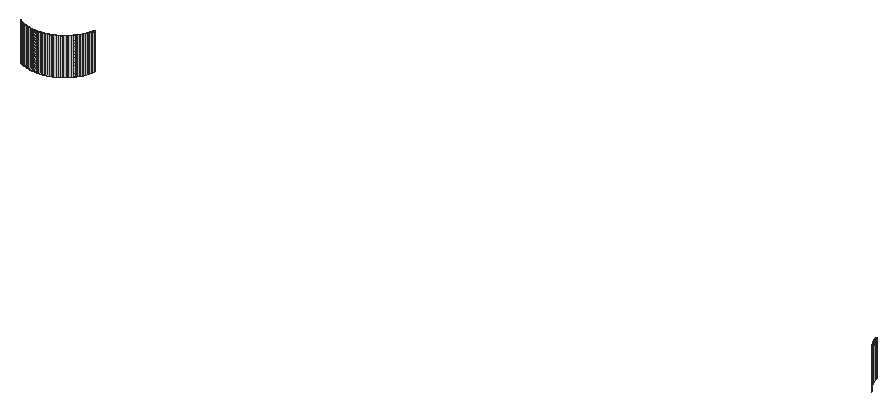
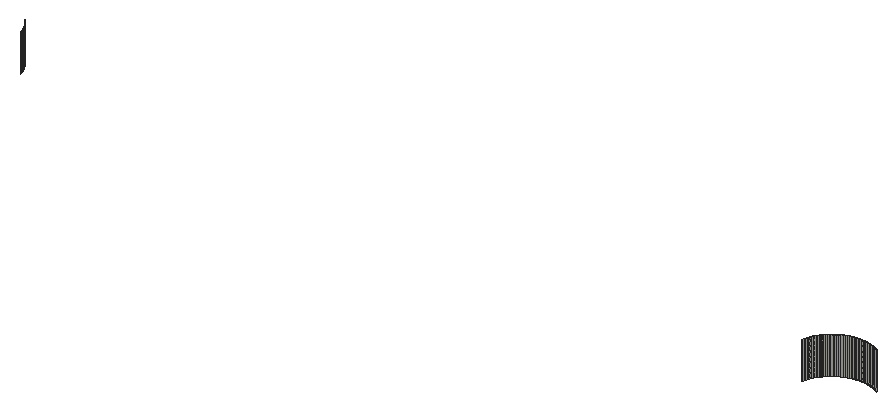
# SketchUp Ruby script. Lengths in inches.
U = 1.inch
M = Sketchup.active_model
def pt(a) = Geom::Point3d.new(a.map { |v| v * U })
def face(e, loops, mat)
  f = e.add_face(loops[0].map { |a| pt(a) })
  loops[1..].each { |l| e.add_face(l.map { |a| pt(a) }).erase! }
  f.material = f.back_material = mat if mat
  f
end
# faces: each face lists its corners as indices into pts; further lists are holes
def faces(e, pts, list, mat = nil) = list.each { |f| face(e, (f[0].is_a?(Array) ? f : [f]).map { |l| l.map { |i| pts[i] } }, mat) }
# xy, xz, yz: faces in a plane at the given z, y or x. An outline is a flat list of corners, or four numbers for a rectangle; further outlines are holes
def ring(l) = l.size == 4 ? [[l[0], l[1]], [l[2], l[1]], [l[2], l[3]], [l[0], l[3]]] : l.each_slice(2).to_a
def flat(e, list, mat, &to3) = list.each { |f| face(e, (f[0].is_a?(Array) ? f : [f]).map { |l| ring(l).map { |u, v| to3.(u, v) } }, mat) }
def xy(e, z, list, mat = nil) = flat(e, list, mat) { |x, y| [x, y, z] }
def xz(e, y, list, mat = nil) = flat(e, list, mat) { |x, z| [x, y, z] }
def yz(e, x, list, mat = nil) = flat(e, list, mat) { |y, z| [x, y, z] }
def lines(e, pts, list) = list.each { |a, b| e.add_line(pt(pts[a]), pt(pts[b])) }
# prism: a flat outline (further loops are holes) pulled along v
def prism(e, loops, v, mat = nil)
  f = face(e, loops, mat); d = Geom::Vector3d.new(v.map { |x| x * U })
  f.pushpull(f.normal.samedirection?(d) ? d.length : -d.length)
end
def box(e, o, s, mat = nil) = prism(e, [[o, [o[0] + s[0], o[1], o[2]], [o[0] + s[0], o[1] + s[1], o[2]], [o[0], o[1] + s[1], o[2]]]], [0, 0, s[2]], mat)
def at(x, y, z, deg = 0) = Geom::Transformation.translation(pt([x, y, z])) * Geom::Transformation.rotation(ORIGIN, Z_AXIS, deg.degrees)
def axes(o, x, y, z) = Geom::Transformation.new([*x, 0, *y, 0, *z, 0, *pt(o).to_a, 1])
def part(name) = M.definitions.add(name)
# library, detail: a bought-in or finely detailed component or shape, given as its bounding box
def library(name, o, s) = part(name).tap { |d| box(d.entities, o, s) }
def detail(e, o, s) = box(e.add_group.entities, o, s)
def put(e, d, t, mat = nil) = e.add_instance(d, t).tap { |i| i.material = mat if mat }
def group(e, t, mat = nil) = e.add_group.tap { |g| g.transformation = t; g.material = mat if mat }.entities
root = M.entities
xz(root,249,[[182.84,348,182.92,351],[182.92,348,183,351],[183,348,183.08,351],[183.08,348,183.16,351]])
p = [[182.53,249.04,348],[182.45,249.05,348],[182.45,249.05,351],[182.53,249.04,351],[182.61,249.03,348],[182.61,249.03,351],
  [182.6875,249.02,348],[182.6875,249.02,351],[182.76,249.01,348],[182.76,249.01,351],[182.84,249,348],[182.84,249,351],
  [183.24,249.01,348],[183.16,249,348],[183.16,249,351],[183.24,249.01,351],[183.3125,249.02,348],[183.3125,249.02,351],
  [183.39,249.03,348],[183.39,249.03,351],[183.47,249.04,348],[183.47,249.04,351],[183.55,249.05,348],[183.55,249.05,351],
  [182.07,249.15,348],[182,249.17,348],[182,249.17,351],[182.07,249.15,351],[182.15,249.125,348],[182.15,249.125,351],
  [182.22,249.1,348],[182.22,249.1,351],[182.3,249.08,348],[182.3,249.08,351],[182.375,249.07,348],[182.375,249.07,351],
  [183.625,249.07,348],[183.625,249.07,351],[183.7,249.08,348],[183.7,249.08,351],[183.78,249.1,348],[183.78,249.1,351],
  [183.85,249.125,348],[183.85,249.125,351],[183.93,249.15,348],[183.93,249.15,351],[184,249.17,348],[184,249.17,351],
  [181.85,249.23,348],[181.78,249.26,348],[181.78,249.26,351],[181.85,249.23,351],[181.92,249.2,348],[181.92,249.2,351],
  [184.07,249.2,348],[184.07,249.2,351],[184.15,249.23,348],[184.15,249.23,351],[184.22,249.26,348],[184.22,249.26,351],
  [181.64,249.33,348],[181.57,249.36,348],[181.57,249.36,351],[181.64,249.33,351],[181.71,249.29,348],[181.71,249.29,351],
  [184.29,249.29,348],[184.29,249.29,351],[184.36,249.33,348],[184.36,249.33,351],[184.43,249.36,348],[184.43,249.36,351],
  [181.5,249.4,348],[181.43,249.44,348],[181.43,249.44,351],[181.5,249.4,351],[184.5,249.4,348],[184.5,249.4,351],
  [184.57,249.44,348],[184.57,249.44,351],[184.63,249.48,348],[184.63,249.48,351],[184.7,249.53,348],[184.7,249.53,351],
  [184.76,249.57,348],[184.76,249.57,351],[184.83,249.62,348],[184.83,249.62,351],[184.89,249.67,348],[184.89,249.67,351],
  [184.95,249.72,348],[184.95,249.72,351],[185.01,249.77,348],[185.01,249.77,351],[185.06,249.82,348],[185.06,249.82,351],
  [185.12,249.88,348],[185.12,249.88,351],[185.18,249.93,348],[185.18,249.93,351],[185.23,249.99,348],[185.23,249.99,351],
  [249.82,249.94,348],[249.77,249.99,348],[249.77,249.99,351],[249.82,249.94,351],[249.88,249.88,348],[249.88,249.88,351],
  [185.28,250.05,348],[185.28,250.05,351],[249.72,250.05,348],[249.72,250.05,351],[185.33,250.11,348],[185.33,250.11,351],
  [185.38,250.17,348],[185.38,250.17,351],[249.67,250.11,348],[249.62,250.17,348],[249.62,250.17,351],[249.67,250.11,351],
  [185.43,250.24,348],[185.43,250.24,351],[185.47,250.3,348],[185.47,250.3,351],[249.57,250.24,348],[249.53,250.3,348],
  [249.53,250.3,351],[249.57,250.24,351],[185.52,250.37,348],[185.52,250.37,351],[249.48,250.37,348],[249.48,250.37,351],
  [185.56,250.43,348],[185.56,250.43,351],[185.6,250.5,348],[185.6,250.5,351],[249.44,250.43,348],[249.4,250.5,348],
  [249.4,250.5,351],[249.44,250.43,351],[185.64,250.57,348],[185.64,250.57,351],[249.36,250.57,348],[249.36,250.57,351],
  [185.67,250.64,348],[185.67,250.64,351],[185.71,250.71,348],[185.71,250.71,351],[249.33,250.64,348],[249.29,250.71,348],
  [249.29,250.71,351],[249.33,250.64,351],[185.74,250.78,348],[185.74,250.78,351],[249.26,250.78,348],[249.26,250.78,351],
  [185.77,250.85,348],[185.77,250.85,351],[249.23,250.85,348],[249.23,250.85,351],[185.8,250.92,348],[185.8,250.92,351],
  [185.83,251,348],[185.83,251,351],[249.2,250.93,348],[249.17,251,348],[249.17,251,351],[249.2,250.93,351],
  [185.85,251.07,348],[185.85,251.07,351],[249.15,251.07,348],[249.15,251.07,351],[185.875,251.15,348],[185.875,251.15,351],
  [185.9,251.22,348],[185.9,251.22,351],[249.125,251.15,348],[249.1,251.22,348],[249.1,251.22,351],[249.125,251.15,351],
  [185.92,251.3,348],[185.92,251.3,351],[249.08,251.3,348],[249.08,251.3,351],[185.93,251.375,348],[185.93,251.375,351]]
faces(root,p,[[0,1,2,3],[4,0,3,5],[6,4,5,7],[8,6,7,9],[10,8,9,11],[12,13,14,15],[16,12,15,17],[18,16,17,19],
  [20,18,19,21],[22,20,21,23],[24,25,26,27],[28,24,27,29],[30,28,29,31],[32,30,31,33],[34,32,33,35],[1,34,35,2],
  [36,22,23,37],[38,36,37,39],[40,38,39,41],[42,40,41,43],[44,42,43,45],[46,44,45,47],[48,49,50,51],[52,48,51,53],
  [25,52,53,26],[54,46,47,55],[56,54,55,57],[58,56,57,59],[60,61,62,63],[64,60,63,65],[49,64,65,50],[66,58,59,67],
  [68,66,67,69],[70,68,69,71],[72,73,74,75],[61,72,75,62],[76,70,71,77],[78,76,77,79],[80,78,79,81],[82,80,81,83],
  [84,82,83,85],[86,84,85,87],[88,86,87,89],[90,88,89,91],[92,90,91,93],[94,92,93,95],[96,94,95,97],[98,96,97,99],
  [100,98,99,101],[102,103,104,105],[106,102,105,107],[108,100,101,109],[103,110,111,104],[112,108,109,113],[114,112,113,115],[116,117,118,119],
  [110,116,119,111],[120,114,115,121],[122,120,121,123],[124,125,126,127],[117,124,127,118],[128,122,123,129],[125,130,131,126],[132,128,129,133],
  [134,132,133,135],[136,137,138,139],[130,136,139,131],[140,134,135,141],[137,142,143,138],[144,140,141,145],[146,144,145,147],[148,149,150,151],
  [142,148,151,143],[152,146,147,153],[149,154,155,150],[156,152,153,157],[154,158,159,155],[160,156,157,161],[162,160,161,163],[164,165,166,167],
  [158,164,167,159],[168,162,163,169],[165,170,171,166],[172,168,169,173],[174,172,173,175],[176,177,178,179],[170,176,179,171],[180,174,175,181],
  [177,182,183,178],[184,180,181,185]])
